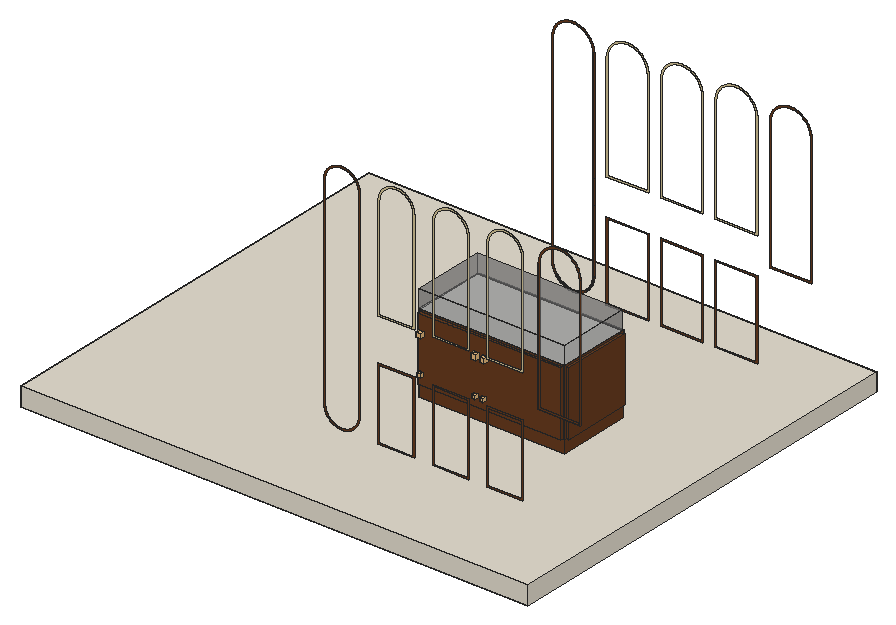
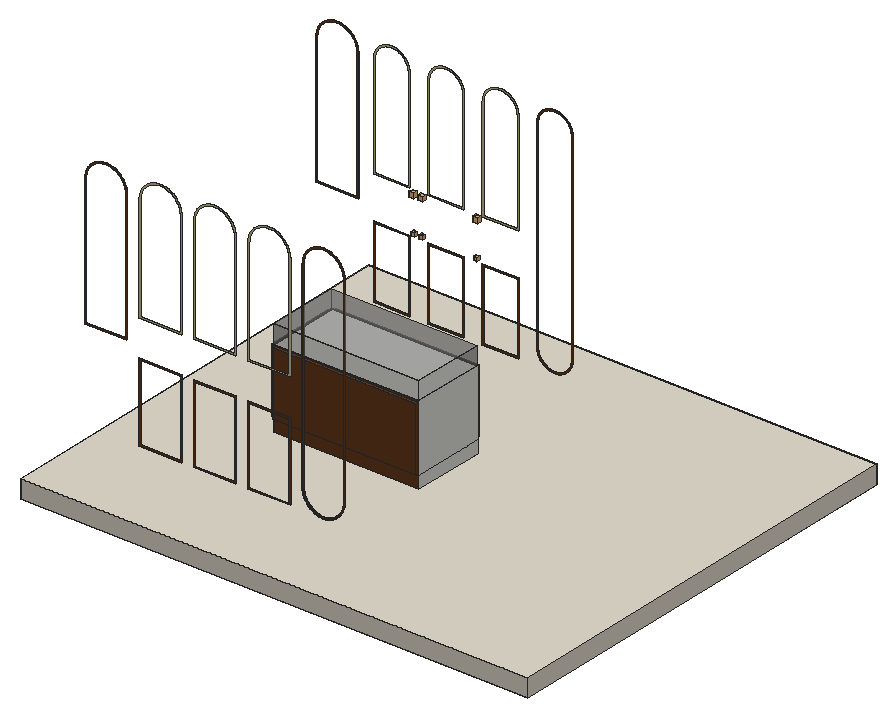
# SketchUp Ruby script. Lengths in inches.
U = 1.inch
M = Sketchup.active_model
def pt(a) = Geom::Point3d.new(a.map { |v| v * U })
def face(e, loops, mat)
  f = e.add_face(loops[0].map { |a| pt(a) })
  loops[1..].each { |l| e.add_face(l.map { |a| pt(a) }).erase! }
  f.material = f.back_material = mat if mat
  f
end
# faces: each face lists its corners as indices into pts; further lists are holes
def faces(e, pts, list, mat = nil) = list.each { |f| face(e, (f[0].is_a?(Array) ? f : [f]).map { |l| l.map { |i| pts[i] } }, mat) }
# xy, xz, yz: faces in a plane at the given z, y or x. An outline is a flat list of corners, or four numbers for a rectangle; further outlines are holes
def ring(l) = l.size == 4 ? [[l[0], l[1]], [l[2], l[1]], [l[2], l[3]], [l[0], l[3]]] : l.each_slice(2).to_a
def flat(e, list, mat, &to3) = list.each { |f| face(e, (f[0].is_a?(Array) ? f : [f]).map { |l| ring(l).map { |u, v| to3.(u, v) } }, mat) }
def xy(e, z, list, mat = nil) = flat(e, list, mat) { |x, y| [x, y, z] }
def xz(e, y, list, mat = nil) = flat(e, list, mat) { |x, z| [x, y, z] }
def yz(e, x, list, mat = nil) = flat(e, list, mat) { |y, z| [x, y, z] }
def lines(e, pts, list) = list.each { |a, b| e.add_line(pt(pts[a]), pt(pts[b])) }
# prism: a flat outline (further loops are holes) pulled along v
def prism(e, loops, v, mat = nil)
  f = face(e, loops, mat); d = Geom::Vector3d.new(v.map { |x| x * U })
  f.pushpull(f.normal.samedirection?(d) ? d.length : -d.length)
end
def box(e, o, s, mat = nil) = prism(e, [[o, [o[0] + s[0], o[1], o[2]], [o[0] + s[0], o[1] + s[1], o[2]], [o[0], o[1] + s[1], o[2]]]], [0, 0, s[2]], mat)
def at(x, y, z, deg = 0) = Geom::Transformation.translation(pt([x, y, z])) * Geom::Transformation.rotation(ORIGIN, Z_AXIS, deg.degrees)
def axes(o, x, y, z) = Geom::Transformation.new([*x, 0, *y, 0, *z, 0, *pt(o).to_a, 1])
def part(name) = M.definitions.add(name)
# library, detail: a bought-in or finely detailed component or shape, given as its bounding box
def library(name, o, s) = part(name).tap { |d| box(d.entities, o, s) }
def detail(e, o, s) = box(e.add_group.entities, o, s)
def put(e, d, t, mat = nil) = e.add_instance(d, t).tap { |i| i.material = mat if mat }
def group(e, t, mat = nil) = e.add_group.tap { |g| g.transformation = t; g.material = mat if mat }.entities
root = M.entities
M.materials.add("138_plaster painted wall texture-seamless").color = [214, 198, 153]
M.materials.add("[Translucent Glass Gray]1").color = [128, 128, 128]
M.materials["[Translucent Glass Gray]1"].alpha = 0.5
M.materials.add("[Wood Veneer 01]").color = [104, 60, 32]
M.materials.add("download (3)").color = [228, 221, 207]
c1 = library("Group\#17",[0,0,0],[1.625,1.625,1.31])
xy(root,36,[[152,24,166,24.2]],"[Wood Veneer 01]")
xz(root,24.2,[[[99,45,99,79,99.01,79.35,99.04,79.7,99.09,80.04,99.16,80.38,99.25,80.72,99.36,81.05,99.49,81.375,99.64,81.69,99.8,82,99.99,82.3,100.1875,82.58,100.4,82.86,100.64,83.12,100.88,83.36,101.14,83.6,101.42,83.8125,101.7,84.01,102,84.2,102.31,84.36,102.625,84.51,102.95,84.64,103.28,84.75,103.62,84.84,103.96,84.91,104.3,84.96,104.65,84.99,105,85,105.35,84.99,105.7,84.96,106.04,84.91,106.38,84.84,106.72,84.75,107.05,84.64,107.375,84.51,107.69,84.36,108,84.2,108.3,84.01,108.58,83.8125,108.86,83.6,109.12,83.36,109.36,83.12,109.6,82.86,109.8125,82.58,110.01,82.3,110.2,82,110.36,81.69,110.51,81.375,110.64,81.05,110.75,80.72,110.84,80.38,110.91,80.04,110.96,79.7,110.99,79.35,111,79,111,45],[99.4,45.4,110.6,45.4,110.6,79,110.59,79.33,110.5625,79.65,110.51,79.97,110.45,80.29,110.36,80.61,110.26,80.92,110.14,81.22,110,81.51,109.85,81.8,109.68,82.08,109.49,82.34,109.29,82.6,109.07,82.84,108.84,83.07,108.6,83.29,108.34,83.49,108.08,83.68,107.8,83.85,107.51,84,107.22,84.14,106.92,84.26,106.61,84.36,106.29,84.45,105.97,84.51,105.65,84.5625,105.33,84.59,105,84.6,104.67,84.59,104.35,84.5625,104.03,84.51,103.71,84.45,103.39,84.36,103.08,84.26,102.78,84.14,102.49,84,102.2,83.85,101.92,83.68,101.66,83.49,101.4,83.29,101.16,83.07,100.93,82.84,100.71,82.6,100.51,82.34,100.32,82.08,100.15,81.8,100,81.51,99.86,81.22,99.74,80.92,99.64,80.61,99.55,80.29,99.49,79.97,99.4375,79.65,99.41,79.33,99.4,79]],[[117,45,117,79,117.01,79.35,117.04,79.7,117.09,80.04,117.16,80.38,117.25,80.72,117.36,81.05,117.49,81.375,117.64,81.69,117.8,82,117.99,82.3,118.1875,82.58,118.4,82.86,118.64,83.12,118.88,83.36,119.14,83.6,119.42,83.8125,119.7,84.01,120,84.2,120.31,84.36,120.625,84.51,120.95,84.64,121.28,84.75,121.62,84.84,121.96,84.91,122.3,84.96,122.65,84.99,123,85,123.35,84.99,123.7,84.96,124.04,84.91,124.38,84.84,124.72,84.75,125.05,84.64,125.375,84.51,125.69,84.36,126,84.2,126.3,84.01,126.58,83.8125,126.86,83.6,127.12,83.36,127.36,83.12,127.6,82.86,127.8125,82.58,128.01,82.3,128.2,82,128.36,81.69,128.51,81.375,128.64,81.05,128.75,80.72,128.84,80.38,128.91,80.04,128.96,79.7,128.99,79.35,129,79,129,45],[117.4,45.4,128.6,45.4,128.6,79,128.59,79.33,128.5625,79.65,128.51,79.97,128.45,80.29,128.36,80.61,128.26,80.92,128.14,81.22,128,81.51,127.85,81.8,127.68,82.08,127.49,82.34,127.29,82.6,127.07,82.84,126.84,83.07,126.6,83.29,126.34,83.49,126.08,83.68,125.8,83.85,125.51,84,125.22,84.14,124.92,84.26,124.61,84.36,124.29,84.45,123.97,84.51,123.65,84.5625,123.33,84.59,123,84.6,122.67,84.59,122.35,84.5625,122.03,84.51,121.71,84.45,121.39,84.36,121.08,84.26,120.78,84.14,120.49,84,120.2,83.85,119.92,83.68,119.66,83.49,119.4,83.29,119.16,83.07,118.93,82.84,118.71,82.6,118.51,82.34,118.32,82.08,118.15,81.8,118,81.51,117.86,81.22,117.74,80.92,117.64,80.61,117.55,80.29,117.49,79.97,117.4375,79.65,117.41,79.33,117.4,79]],[[135,45,135,79,135.01,79.35,135.04,79.7,135.09,80.04,135.16,80.38,135.25,80.72,135.36,81.05,135.49,81.375,135.64,81.69,135.8,82,135.99,82.3,136.1875,82.58,136.4,82.86,136.64,83.12,136.88,83.36,137.14,83.6,137.42,83.8125,137.7,84.01,138,84.2,138.31,84.36,138.625,84.51,138.95,84.64,139.28,84.75,139.62,84.84,139.96,84.91,140.3,84.96,140.65,84.99,141,85,141.35,84.99,141.7,84.96,142.04,84.91,142.38,84.84,142.72,84.75,143.05,84.64,143.375,84.51,143.69,84.36,144,84.2,144.3,84.01,144.58,83.8125,144.86,83.6,145.12,83.36,145.36,83.12,145.6,82.86,145.8125,82.58,146.01,82.3,146.2,82,146.36,81.69,146.51,81.375,146.64,81.05,146.75,80.72,146.84,80.38,146.91,80.04,146.96,79.7,146.99,79.35,147,79,147,45],[135.4,45.4,146.6,45.4,146.6,79,146.59,79.33,146.5625,79.65,146.51,79.97,146.45,80.29,146.36,80.61,146.26,80.92,146.14,81.22,146,81.51,145.85,81.8,145.68,82.08,145.49,82.34,145.29,82.6,145.07,82.84,144.84,83.07,144.6,83.29,144.34,83.49,144.08,83.68,143.8,83.85,143.51,84,143.22,84.14,142.92,84.26,142.61,84.36,142.29,84.45,141.97,84.51,141.65,84.5625,141.33,84.59,141,84.6,140.67,84.59,140.35,84.5625,140.03,84.51,139.71,84.45,139.39,84.36,139.08,84.26,138.78,84.14,138.49,84,138.2,83.85,137.92,83.68,137.66,83.49,137.4,83.29,137.16,83.07,136.93,82.84,136.71,82.6,136.51,82.34,136.32,82.08,136.15,81.8,136,81.51,135.86,81.22,135.74,80.92,135.64,80.61,135.55,80.29,135.49,79.97,135.4375,79.65,135.41,79.33,135.4,79]]],"138_plaster painted wall texture-seamless")
xz(root,24.2,[[[87,7,86.65,7.01,86.3,7.04,85.96,7.09,85.62,7.16,85.28,7.25,84.95,7.36,84.625,7.49,84.31,7.64,84,7.8,83.7,7.99,83.42,8.1875,83.14,8.4,82.88,8.64,82.64,8.88,82.4,9.14,82.1875,9.42,81.99,9.7,81.8,10,81.64,10.31,81.49,10.625,81.36,10.95,81.25,11.28,81.16,11.62,81.09,11.96,81.04,12.3,81.01,12.65,81,13,81,79,81.01,79.35,81.04,79.7,81.09,80.04,81.16,80.38,81.25,80.72,81.36,81.05,81.49,81.375,81.64,81.69,81.8,82,81.99,82.3,82.1875,82.58,82.4,82.86,82.64,83.12,82.88,83.36,83.14,83.6,83.42,83.8125,83.7,84.01,84,84.2,84.31,84.36,84.625,84.51,84.95,84.64,85.28,84.75,85.62,84.84,85.96,84.91,86.3,84.96,86.65,84.99,87,85,87.35,84.99,87.7,84.96,88.04,84.91,88.38,84.84,88.72,84.75,89.05,84.64,89.375,84.51,89.69,84.36,90,84.2,90.3,84.01,90.58,83.8125,90.86,83.6,91.12,83.36,91.36,83.12,91.6,82.86,91.8125,82.58,92.01,82.3,92.2,82,92.36,81.69,92.51,81.375,92.64,81.05,92.75,80.72,92.84,80.38,92.91,80.04,92.96,79.7,92.99,79.35,93,79,93,13,92.99,12.65,92.96,12.3,92.91,11.96,92.84,11.62,92.75,11.28,92.64,10.95,92.51,10.625,92.36,10.31,92.2,10,92.01,9.7,91.8125,9.42,91.6,9.14,91.36,8.88,91.12,8.64,90.86,8.4,90.58,8.1875,90.3,7.99,90,7.8,89.69,7.64,89.375,7.49,89.05,7.36,88.72,7.25,88.38,7.16,88.04,7.09,87.7,7.04,87.35,7.01],[87,7.4,87.33,7.41,87.65,7.4375,87.97,7.49,88.29,7.55,88.61,7.64,88.92,7.74,89.22,7.86,89.51,8,89.8,8.15,90.08,8.32,90.34,8.51,90.6,8.71,90.84,8.93,91.07,9.16,91.29,9.4,91.49,9.66,91.68,9.92,91.85,10.2,92,10.49,92.14,10.78,92.26,11.08,92.36,11.39,92.45,11.71,92.51,12.03,92.5625,12.35,92.59,12.67,92.6,13,92.6,79,92.59,79.33,92.5625,79.65,92.51,79.97,92.45,80.29,92.36,80.61,92.26,80.92,92.14,81.22,92,81.51,91.85,81.8,91.68,82.08,91.49,82.34,91.29,82.6,91.07,82.84,90.84,83.07,90.6,83.29,90.34,83.49,90.08,83.68,89.8,83.85,89.51,84,89.22,84.14,88.92,84.26,88.61,84.36,88.29,84.45,87.97,84.51,87.65,84.5625,87.33,84.59,87,84.6,86.67,84.59,86.35,84.5625,86.03,84.51,85.71,84.45,85.39,84.36,85.08,84.26,84.78,84.14,84.49,84,84.2,83.85,83.92,83.68,83.66,83.49,83.4,83.29,83.16,83.07,82.93,82.84,82.71,82.6,82.51,82.34,82.32,82.08,82.15,81.8,82,81.51,81.86,81.22,81.74,80.92,81.64,80.61,81.55,80.29,81.49,79.97,81.4375,79.65,81.41,79.33,81.4,79,81.4,13,81.41,12.67,81.4375,12.35,81.49,12.03,81.55,11.71,81.64,11.39,81.74,11.08,81.86,10.78,82,10.49,82.15,10.2,82.32,9.92,82.51,9.66,82.71,9.4,82.93,9.16,83.16,8.93,83.4,8.71,83.66,8.51,83.92,8.32,84.2,8.15,84.49,8,84.78,7.86,85.08,7.74,85.39,7.64,85.71,7.55,86.03,7.49,86.35,7.4375,86.67,7.41]],[[99,7,111,31],[99.4,7.4,110.6,30.6]],[[117,7,129,31],[117.4,7.4,128.6,30.6]],[[135,7,147,31],[135.4,7.4,146.6,30.6]],[[152,36,152,79,152.01,79.41,152.05,79.8125,152.11,80.22,152.1875,80.61,152.29,81.01,152.42,81.39,152.57,81.77,152.74,82.14,152.9375,82.5,153.15,82.85,153.39,83.18,153.64,83.5,153.91,83.8,154.2,84.09,154.5,84.36,154.82,84.61,155.15,84.85,155.5,85.0625,155.86,85.26,156.23,85.43,156.61,85.58,156.99,85.71,157.39,85.8125,157.78,85.89,158.1875,85.95,158.59,85.99,159,86,159.41,85.99,159.8125,85.95,160.22,85.89,160.61,85.8125,161.01,85.71,161.39,85.58,161.77,85.43,162.14,85.26,162.5,85.0625,162.85,84.85,163.18,84.61,163.5,84.36,163.8,84.09,164.09,83.8,164.36,83.5,164.61,83.18,164.85,82.85,165.0625,82.5,165.26,82.14,165.43,81.77,165.58,81.39,165.71,81.01,165.8125,80.61,165.89,80.22,165.95,79.8125,165.99,79.41,166,79,166,36],[152.4,36.4,165.6,36.4,165.6,79,165.59,79.38,165.56,79.77,165.5,80.15,165.42,80.52,165.32,80.89,165.2,81.26,165.06,81.61,164.9,81.96,164.72,82.3,164.51,82.625,164.29,82.94,164.06,83.24,163.8,83.53,163.53,83.8,163.24,84.06,162.94,84.29,162.625,84.51,162.3,84.72,161.96,84.9,161.61,85.06,161.26,85.2,160.89,85.32,160.52,85.42,160.15,85.5,159.77,85.56,159.38,85.59,159,85.6,158.62,85.59,158.23,85.56,157.85,85.5,157.48,85.42,157.11,85.32,156.74,85.2,156.39,85.06,156.04,84.9,155.7,84.72,155.375,84.51,155.06,84.29,154.76,84.06,154.47,83.8,154.2,83.53,153.94,83.24,153.71,82.94,153.49,82.625,153.28,82.3,153.1,81.96,152.94,81.61,152.8,81.26,152.68,80.89,152.58,80.52,152.5,80.15,152.44,79.77,152.41,79.38,152.4,79]]],"[Wood Veneer 01]")
xz(root,119.8,[[[98,44,112,44,112,79,111.99,79.46,111.94,79.91,111.87,80.37,111.76,80.8125,111.63,81.25,111.47,81.68,111.28,82.1,111.0625,82.5,110.82,82.89,110.55,83.26,110.26,83.62,109.95,83.95,109.62,84.26,109.26,84.55,108.89,84.82,108.5,85.0625,108.1,85.28,107.68,85.47,107.25,85.63,106.8125,85.76,106.37,85.87,105.91,85.94,105.46,85.99,105,86,104.54,85.99,104.09,85.94,103.63,85.87,103.1875,85.76,102.75,85.63,102.32,85.47,101.9,85.28,101.5,85.0625,101.11,84.82,100.74,84.55,100.38,84.26,100.05,83.95,99.74,83.62,99.45,83.26,99.18,82.89,98.9375,82.5,98.72,82.1,98.53,81.68,98.37,81.25,98.24,80.8125,98.13,80.37,98.06,79.91,98.01,79.46,98,79],[98.4,44.4,98.4,79,98.41,79.43,98.46,79.86,98.53,80.29,98.625,80.71,98.75,81.12,98.9,81.53,99.08,81.92,99.28,82.3,99.51,82.67,99.76,83.02,100.04,83.35,100.33,83.67,100.65,83.96,100.98,84.24,101.33,84.49,101.7,84.72,102.08,84.92,102.47,85.1,102.88,85.25,103.29,85.375,103.71,85.47,104.14,85.54,104.57,85.59,105,85.6,105.43,85.59,105.86,85.54,106.29,85.47,106.71,85.375,107.12,85.25,107.53,85.1,107.92,84.92,108.3,84.72,108.67,84.49,109.02,84.24,109.35,83.96,109.67,83.67,109.96,83.35,110.24,83.02,110.49,82.67,110.72,82.3,110.92,81.92,111.1,81.53,111.25,81.12,111.375,80.71,111.47,80.29,111.54,79.86,111.59,79.43,111.6,79,111.6,44.4]],[[116,44,130,44,130,79,129.99,79.46,129.94,79.91,129.87,80.37,129.76,80.8125,129.63,81.25,129.47,81.68,129.28,82.1,129.0625,82.5,128.82,82.89,128.55,83.26,128.26,83.62,127.95,83.95,127.62,84.26,127.26,84.55,126.89,84.82,126.5,85.0625,126.1,85.28,125.68,85.47,125.25,85.63,124.8125,85.76,124.37,85.87,123.91,85.94,123.46,85.99,123,86,122.54,85.99,122.09,85.94,121.63,85.87,121.1875,85.76,120.75,85.63,120.32,85.47,119.9,85.28,119.5,85.0625,119.11,84.82,118.74,84.55,118.38,84.26,118.05,83.95,117.74,83.62,117.45,83.26,117.18,82.89,116.9375,82.5,116.72,82.1,116.53,81.68,116.37,81.25,116.24,80.8125,116.13,80.37,116.06,79.91,116.01,79.46,116,79],[116.4,44.4,116.4,79,116.41,79.43,116.46,79.86,116.53,80.29,116.625,80.71,116.75,81.12,116.9,81.53,117.08,81.92,117.28,82.3,117.51,82.67,117.76,83.02,118.04,83.35,118.33,83.67,118.65,83.96,118.98,84.24,119.33,84.49,119.7,84.72,120.08,84.92,120.47,85.1,120.88,85.25,121.29,85.375,121.71,85.47,122.14,85.54,122.57,85.59,123,85.6,123.43,85.59,123.86,85.54,124.29,85.47,124.71,85.375,125.12,85.25,125.53,85.1,125.92,84.92,126.3,84.72,126.67,84.49,127.02,84.24,127.35,83.96,127.67,83.67,127.96,83.35,128.24,83.02,128.49,82.67,128.72,82.3,128.92,81.92,129.1,81.53,129.25,81.12,129.375,80.71,129.47,80.29,129.54,79.86,129.59,79.43,129.6,79,129.6,44.4]],[[134,44,148,44,148,79,147.99,79.46,147.94,79.91,147.87,80.37,147.76,80.8125,147.63,81.25,147.47,81.68,147.28,82.1,147.0625,82.5,146.82,82.89,146.55,83.26,146.26,83.62,145.95,83.95,145.62,84.26,145.26,84.55,144.89,84.82,144.5,85.0625,144.1,85.28,143.68,85.47,143.25,85.63,142.8125,85.76,142.37,85.87,141.91,85.94,141.46,85.99,141,86,140.54,85.99,140.09,85.94,139.63,85.87,139.1875,85.76,138.75,85.63,138.32,85.47,137.9,85.28,137.5,85.0625,137.11,84.82,136.74,84.55,136.38,84.26,136.05,83.95,135.74,83.62,135.45,83.26,135.18,82.89,134.9375,82.5,134.72,82.1,134.53,81.68,134.37,81.25,134.24,80.8125,134.13,80.37,134.06,79.91,134.01,79.46,134,79],[134.4,44.4,134.4,79,134.41,79.43,134.46,79.86,134.53,80.29,134.625,80.71,134.75,81.12,134.9,81.53,135.08,81.92,135.28,82.3,135.51,82.67,135.76,83.02,136.04,83.35,136.33,83.67,136.65,83.96,136.98,84.24,137.33,84.49,137.7,84.72,138.08,84.92,138.47,85.1,138.88,85.25,139.29,85.375,139.71,85.47,140.14,85.54,140.57,85.59,141,85.6,141.43,85.59,141.86,85.54,142.29,85.47,142.71,85.375,143.12,85.25,143.53,85.1,143.92,84.92,144.3,84.72,144.67,84.49,145.02,84.24,145.35,83.96,145.67,83.67,145.96,83.35,146.24,83.02,146.49,82.67,146.72,82.3,146.92,81.92,147.1,81.53,147.25,81.12,147.375,80.71,147.47,80.29,147.54,79.86,147.59,79.43,147.6,79,147.6,44.4]]],"138_plaster painted wall texture-seamless")
xz(root,119.8,[[[87,6,87.46,6.01,87.91,6.06,88.37,6.13,88.8125,6.24,89.25,6.37,89.68,6.53,90.1,6.72,90.5,6.9375,90.89,7.18,91.26,7.45,91.62,7.74,91.95,8.05,92.26,8.38,92.55,8.74,92.82,9.11,93.0625,9.5,93.28,9.9,93.47,10.32,93.63,10.75,93.76,11.1875,93.87,11.63,93.94,12.09,93.99,12.54,94,13,94,79,93.99,79.46,93.94,79.91,93.87,80.37,93.76,80.8125,93.63,81.25,93.47,81.68,93.28,82.1,93.0625,82.5,92.82,82.89,92.55,83.26,92.26,83.62,91.95,83.95,91.62,84.26,91.26,84.55,90.89,84.82,90.5,85.0625,90.1,85.28,89.68,85.47,89.25,85.63,88.8125,85.76,88.37,85.87,87.91,85.94,87.46,85.99,87,86,86.54,85.99,86.09,85.94,85.63,85.87,85.1875,85.76,84.75,85.63,84.32,85.47,83.9,85.28,83.5,85.0625,83.11,84.82,82.74,84.55,82.38,84.26,82.05,83.95,81.74,83.62,81.45,83.26,81.18,82.89,80.9375,82.5,80.72,82.1,80.53,81.68,80.37,81.25,80.24,80.8125,80.13,80.37,80.06,79.91,80.01,79.46,80,79,80,13,80.01,12.54,80.06,12.09,80.13,11.63,80.24,11.1875,80.37,10.75,80.53,10.32,80.72,9.9,80.9375,9.5,81.18,9.11,81.45,8.74,81.74,8.38,82.05,8.05,82.38,7.74,82.74,7.45,83.11,7.18,83.5,6.9375,83.9,6.72,84.32,6.53,84.75,6.37,85.1875,6.24,85.63,6.13,86.09,6.06,86.54,6.01],[87,6.4,86.57,6.41,86.14,6.46,85.71,6.53,85.29,6.625,84.88,6.75,84.47,6.9,84.08,7.08,83.7,7.28,83.33,7.51,82.98,7.76,82.65,8.04,82.33,8.33,82.04,8.65,81.76,8.98,81.51,9.33,81.28,9.7,81.08,10.08,80.9,10.47,80.75,10.88,80.625,11.29,80.53,11.71,80.46,12.14,80.41,12.57,80.4,13,80.4,79,80.41,79.43,80.46,79.86,80.53,80.29,80.625,80.71,80.75,81.12,80.9,81.53,81.08,81.92,81.28,82.3,81.51,82.67,81.76,83.02,82.04,83.35,82.33,83.67,82.65,83.96,82.98,84.24,83.33,84.49,83.7,84.72,84.08,84.92,84.47,85.1,84.88,85.25,85.29,85.375,85.71,85.47,86.14,85.54,86.57,85.59,87,85.6,87.43,85.59,87.86,85.54,88.29,85.47,88.71,85.375,89.12,85.25,89.53,85.1,89.92,84.92,90.3,84.72,90.67,84.49,91.02,84.24,91.35,83.96,91.67,83.67,91.96,83.35,92.24,83.02,92.49,82.67,92.72,82.3,92.92,81.92,93.1,81.53,93.25,81.12,93.375,80.71,93.47,80.29,93.54,79.86,93.59,79.43,93.6,79,93.6,13,93.59,12.57,93.54,12.14,93.47,11.71,93.375,11.29,93.25,10.88,93.1,10.47,92.92,10.08,92.72,9.7,92.49,9.33,92.24,8.98,91.96,8.65,91.67,8.33,91.35,8.04,91.02,7.76,90.67,7.51,90.3,7.28,89.92,7.08,89.53,6.9,89.12,6.75,88.71,6.625,88.29,6.53,87.86,6.46,87.43,6.41]],[[98,6,112,32],[98.4,6.4,111.6,31.6]],[[116,6,130,32],[116.4,6.4,129.6,31.6]],[[134,6,148,32],[134.4,6.4,147.6,31.6]],[[152,36,166,36,166,79,165.99,79.39,165.96,79.77,165.9,80.15,165.83,80.53,165.74,80.9,165.62,81.27,165.49,81.63,165.33,81.99,165.16,82.33,164.96,82.67,164.75,82.99,164.52,83.3,164.28,83.6,164.02,83.88,163.74,84.15,163.45,84.4,163.15,84.64,162.83,84.86,162.5,85.0625,162.16,85.25,161.8125,85.41,161.45,85.56,161.09,85.68,160.72,85.79,160.34,85.87,159.96,85.93,159.58,85.98,159.19,86,158.81,86,158.42,85.98,158.04,85.93,157.66,85.87,157.28,85.79,156.91,85.68,156.55,85.56,156.1875,85.41,155.84,85.25,155.5,85.0625,155.17,84.86,154.85,84.64,154.55,84.4,154.26,84.15,153.98,83.88,153.72,83.6,153.48,83.3,153.25,82.99,153.04,82.67,152.84,82.33,152.67,81.99,152.51,81.63,152.38,81.27,152.26,80.9,152.17,80.53,152.1,80.15,152.04,79.77,152.01,79.39,152,79],[152.4,36.4,152.4,79,152.41,79.36,152.44,79.73,152.49,80.09,152.56,80.44,152.65,80.8,152.76,81.14,152.89,81.48,153.03,81.82,153.2,82.14,153.38,82.46,153.58,82.76,153.79,83.05,154.02,83.33,154.27,83.6,154.53,83.86,154.8,84.09,155.09,84.32,155.39,84.53,155.7,84.72,156.02,84.89,156.35,85.04,156.6875,85.18,157.03,85.3,157.38,85.4,157.73,85.48,158.09,85.54,158.45,85.58,158.82,85.6,159.18,85.6,159.55,85.58,159.91,85.54,160.27,85.48,160.62,85.4,160.97,85.3,161.3125,85.18,161.65,85.04,161.98,84.89,162.3,84.72,162.61,84.53,162.91,84.32,163.2,84.09,163.47,83.86,163.73,83.6,163.98,83.33,164.21,83.05,164.42,82.76,164.62,82.46,164.8,82.14,164.97,81.82,165.11,81.48,165.24,81.14,165.35,80.8,165.44,80.44,165.51,80.09,165.56,79.73,165.59,79.36,165.6,79,165.6,36.4]]],"[Wood Veneer 01]")
yz(root,93.6,[[119.8,13,120,34],[119.8,34,120,42],[119.8,42,120,79]],"[Wood Veneer 01]")
yz(root,94,[[119.8,13,120,34],[119.8,34,120,42],[119.8,42,120,79]],"[Wood Veneer 01]")
yz(root,152,[[24,36,24.2,79]],"[Wood Veneer 01]")
yz(root,166,[[24,36,24.2,79]],"[Wood Veneer 01]")
p = [[86.09,120,6.06],[86.54,120,6.01],[86.54,119.8,6.01],[86.09,119.8,6.06],[87,120,6],[87,119.8,6],
  [87.46,120,6.01],[87.46,119.8,6.01],[87.91,120,6.06],[87.91,119.8,6.06],[85.1875,120,6.24],[85.63,120,6.13],
  [85.63,119.8,6.13],[85.1875,119.8,6.24],[88.37,120,6.13],[88.37,119.8,6.13],[88.8125,120,6.24],[88.8125,119.8,6.24],
  [84.75,120,6.37],[84.75,119.8,6.37],[89.25,120,6.37],[89.25,119.8,6.37],[84.32,120,6.53],[84.32,119.8,6.53],
  [86.57,120,6.41],[86.14,120,6.46],[86.14,119.8,6.46],[86.57,119.8,6.41],[87,120,6.4],[87,119.8,6.4],
  [87.43,120,6.41],[87.43,119.8,6.41],[87.86,120,6.46],[87.86,119.8,6.46],[89.68,120,6.53],[89.68,119.8,6.53],
  [83.9,120,6.72],[83.9,119.8,6.72],[85.71,120,6.53],[85.29,120,6.625],[85.29,119.8,6.625],[85.71,119.8,6.53],
  [88.29,120,6.53],[88.29,119.8,6.53],[88.71,120,6.625],[88.71,119.8,6.625],[90.1,120,6.72],[90.1,119.8,6.72],
  [84.88,120,6.75],[84.88,119.8,6.75],[89.12,120,6.75],[89.12,119.8,6.75],[83.5,120,6.9375],[83.5,119.8,6.9375],
  [90.5,120,6.9375],[90.5,119.8,6.9375],[84.47,120,6.9],[84.47,119.8,6.9],[89.53,120,6.9],[89.53,119.8,6.9],
  [83.11,120,7.18],[83.11,119.8,7.18],[84.08,120,7.08],[84.08,119.8,7.08],[89.92,120,7.08],[89.92,119.8,7.08],
  [90.89,120,7.18],[90.89,119.8,7.18],[83.7,120,7.28],[83.7,119.8,7.28],[90.3,120,7.28],[90.3,119.8,7.28],
  [82.74,120,7.45],[82.74,119.8,7.45],[91.26,120,7.45],[91.26,119.8,7.45],[83.33,120,7.51],[83.33,119.8,7.51],
  [90.67,120,7.51],[90.67,119.8,7.51],[82.38,120,7.74],[82.38,119.8,7.74],[91.62,120,7.74],[91.62,119.8,7.74],
  [82.98,120,7.76],[82.98,119.8,7.76],[91.02,120,7.76],[91.02,119.8,7.76],[82.05,120,8.05],[82.05,119.8,8.05],
  [91.95,120,8.05],[91.95,119.8,8.05],[82.65,120,8.04],[82.65,119.8,8.04],[91.35,120,8.04],[91.35,119.8,8.04],
  [82.33,120,8.33],[82.33,119.8,8.33],[91.67,120,8.33],[91.67,119.8,8.33],[81.74,120,8.38],[81.74,119.8,8.38],
  [92.26,120,8.38],[92.26,119.8,8.38],[82.04,120,8.65],[82.04,119.8,8.65],[91.96,120,8.65],[91.96,119.8,8.65],
  [81.45,120,8.74],[81.45,119.8,8.74],[92.55,120,8.74],[92.55,119.8,8.74],[81.76,120,8.98],[81.76,119.8,8.98],
  [92.24,120,8.98],[92.24,119.8,8.98],[92.82,120,9.11],[92.82,119.8,9.11],[81.51,120,9.33],[81.51,119.8,9.33],
  [92.49,120,9.33],[92.49,119.8,9.33],[93.0625,120,9.5],[93.0625,119.8,9.5],[92.72,120,9.7],[92.72,119.8,9.7],
  [93.28,120,9.9],[93.28,119.8,9.9],[92.92,120,10.08],[92.92,119.8,10.08],[93.47,120,10.32],[93.47,119.8,10.32],
  [93.1,120,10.47],[93.1,119.8,10.47],[93.63,120,10.75],[93.63,119.8,10.75],[93.25,120,10.88],[93.25,119.8,10.88],
  [93.76,120,11.1875],[93.76,119.8,11.1875],[93.375,120,11.29],[93.375,119.8,11.29],[93.87,120,11.63],[93.87,119.8,11.63],
  [93.47,120,11.71],[93.47,119.8,11.71],[93.94,120,12.09],[93.94,119.8,12.09],[93.54,120,12.14],[93.54,119.8,12.14],
  [93.59,120,12.57],[93.59,119.8,12.57],[93.99,120,12.54],[93.99,119.8,12.54],[94,120,13],[94,119.8,13],
  [93.6,120,13],[93.6,119.8,13]]
faces(root,p,[[0,1,2,3],[1,4,5,2],[4,6,7,5],[6,8,9,7],[10,11,12,13],[11,0,3,12],[8,14,15,9],[14,16,17,15],
  [18,10,13,19],[16,20,21,17],[22,18,19,23],[24,25,26,27],[28,24,27,29],[30,28,29,31],[32,30,31,33],[20,34,35,21],
  [36,22,23,37],[38,39,40,41],[25,38,41,26],[42,32,33,43],[44,42,43,45],[34,46,47,35],[39,48,49,40],[50,44,45,51],
  [52,36,37,53],[46,54,55,47],[48,56,57,49],[58,50,51,59],[60,52,53,61],[56,62,63,57],[64,58,59,65],[54,66,67,55],
  [62,68,69,63],[70,64,65,71],[72,60,61,73],[66,74,75,67],[68,76,77,69],[78,70,71,79],[80,72,73,81],[74,82,83,75],
  [76,84,85,77],[86,78,79,87],[88,80,81,89],[82,90,91,83],[84,92,93,85],[94,86,87,95],[92,96,97,93],[98,94,95,99],
  [100,88,89,101],[90,102,103,91],[96,104,105,97],[106,98,99,107],[108,100,101,109],[102,110,111,103],[104,112,113,105],[114,106,107,115],
  [110,116,117,111],[112,118,119,113],[120,114,115,121],[116,122,123,117],[124,120,121,125],[122,126,127,123],[128,124,125,129],[126,130,131,127],
  [132,128,129,133],[130,134,135,131],[136,132,133,137],[134,138,139,135],[140,136,137,141],[138,142,143,139],[144,140,141,145],[142,146,147,143],
  [148,144,145,149],[150,148,149,151],[146,152,153,147],[152,154,155,153],[156,150,151,157]],"[Wood Veneer 01]")
put(root,c1,axes([112.06,24,32.84],[0.75,0,0],[0,0,-0.75],[0,0.75,0]),"[Wood Veneer 01]")
put(root,c1,axes([130.06,24,32.84],[0.75,0,0],[0,0,-0.75],[0,0.75,0]),"[Wood Veneer 01]")
put(root,c1,axes([132.74,24,32.84],[0.75,0,0],[0,0,-0.75],[0,0.75,0]),"[Wood Veneer 01]")
put(root,c1,axes([111.72,24,44.81],[1,0,0],[0,0,-1],[0,1,0]),"[Wood Veneer 01]")
put(root,c1,axes([129.72,24,44.81],[1,0,0],[0,0,-1],[0,1,0]),"[Wood Veneer 01]")
put(root,c1,axes([132.66,24,44.81],[1,0,0],[0,0,-1],[0,1,0]),"[Wood Veneer 01]")
g1 = group(root,at(24,0,-6))
box(g1,[-24,0,0],[168,144,6],"download (3)")
g2 = group(root,at(84,60,0))
xy(g2,0,[[0,0,48,24]])
xy(g2,4,[[0,0,48,24]])
xy(g2,4.4,[[0.4,-1,47.6,0],[48,0.4,49,23.6],[0.4,24,47.6,25]],"[Wood Veneer 01]")
xy(g2,25.6,[[0.4,-1,47.6,0],[48,0.4,49,23.6],[0.4,24,47.6,25]],"[Wood Veneer 01]")
xy(g2,26,[[0,0,48,24]])
xy(g2,32,[[0,0,48,24]],"[Translucent Glass Gray]1")
xz(g2,-1,[[0.4,4.4,47.6,25.6]],"[Wood Veneer 01]")
xz(g2,0,[[0,26,48,32]],"[Translucent Glass Gray]1")
xz(g2,0,[[0,0,48,4],[[0,4,48,26],[0.4,4.4,47.6,25.6]]],"[Wood Veneer 01]")
xz(g2,0.4,[[48,4.4,49,25.6]],"[Wood Veneer 01]")
xz(g2,23.6,[[48,4.4,49,25.6]],"[Wood Veneer 01]")
xz(g2,24,[[0,26,48,32]],"[Translucent Glass Gray]1")
xz(g2,24,[[0,0,48,4],[[0,4,48,26],[0.4,4.4,47.6,25.6]]],"[Wood Veneer 01]")
xz(g2,25,[[0.4,4.4,47.6,25.6]],"[Wood Veneer 01]")
yz(g2,0,[[0,0,24,4],[0,4,24,26]])
yz(g2,0,[[0,26,24,32]],"[Translucent Glass Gray]1")
yz(g2,0.4,[[-1,4.4,0,25.6],[24,4.4,25,25.6]],"[Wood Veneer 01]")
yz(g2,47.6,[[-1,4.4,0,25.6],[24,4.4,25,25.6]],"[Wood Veneer 01]")
yz(g2,48,[[0,26,24,32]],"[Translucent Glass Gray]1")
yz(g2,48,[[0,0,24,4],[[0,4,24,26],[0.4,4.4,23.6,25.6]]],"[Wood Veneer 01]")
yz(g2,49,[[0.4,4.4,23.6,25.6]],"[Wood Veneer 01]")
